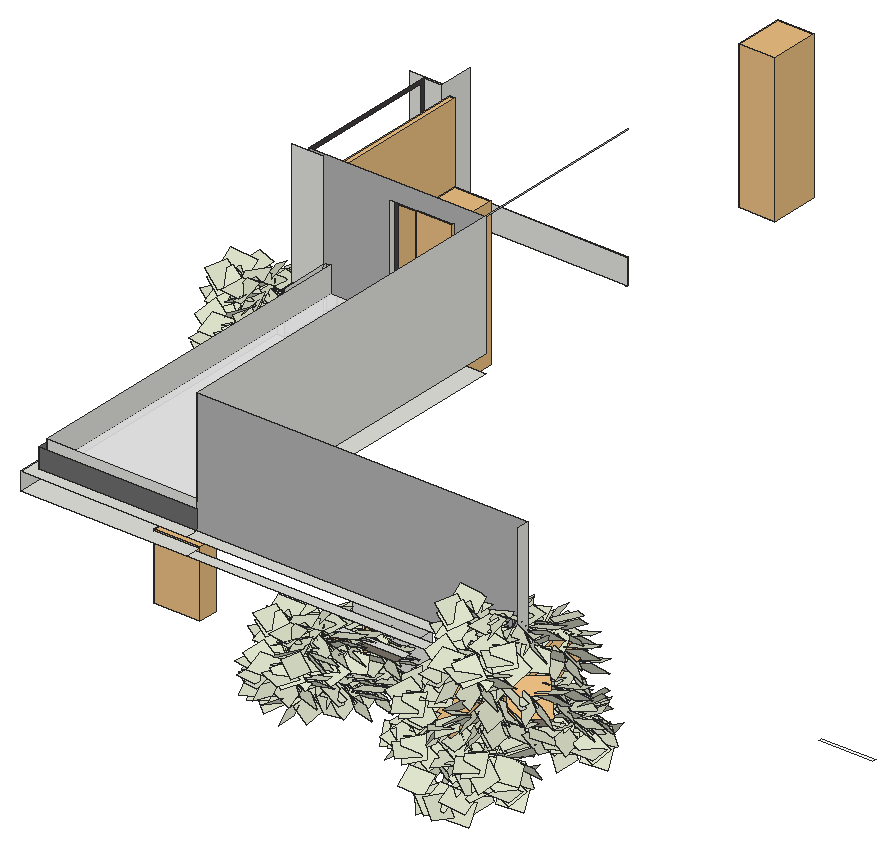
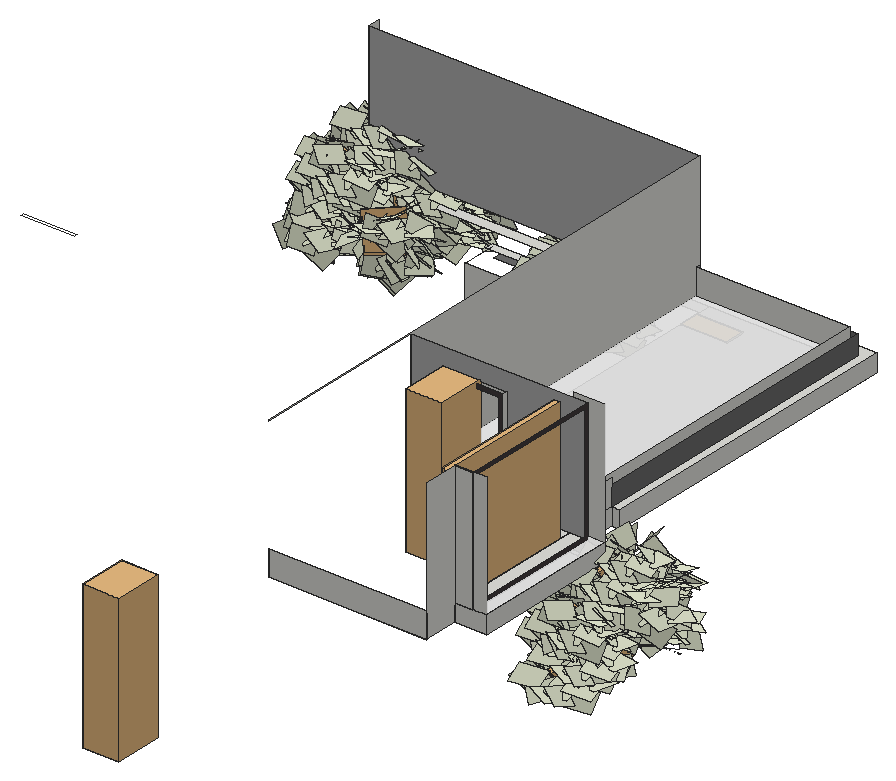
# SketchUp Ruby script. Lengths in inches.
U = 1.inch
M = Sketchup.active_model
def pt(a) = Geom::Point3d.new(a.map { |v| v * U })
def face(e, loops, mat)
  f = e.add_face(loops[0].map { |a| pt(a) })
  loops[1..].each { |l| e.add_face(l.map { |a| pt(a) }).erase! }
  f.material = f.back_material = mat if mat
  f
end
# faces: each face lists its corners as indices into pts; further lists are holes
def faces(e, pts, list, mat = nil) = list.each { |f| face(e, (f[0].is_a?(Array) ? f : [f]).map { |l| l.map { |i| pts[i] } }, mat) }
# xy, xz, yz: faces in a plane at the given z, y or x. An outline is a flat list of corners, or four numbers for a rectangle; further outlines are holes
def ring(l) = l.size == 4 ? [[l[0], l[1]], [l[2], l[1]], [l[2], l[3]], [l[0], l[3]]] : l.each_slice(2).to_a
def flat(e, list, mat, &to3) = list.each { |f| face(e, (f[0].is_a?(Array) ? f : [f]).map { |l| ring(l).map { |u, v| to3.(u, v) } }, mat) }
def xy(e, z, list, mat = nil) = flat(e, list, mat) { |x, y| [x, y, z] }
def xz(e, y, list, mat = nil) = flat(e, list, mat) { |x, z| [x, y, z] }
def yz(e, x, list, mat = nil) = flat(e, list, mat) { |y, z| [x, y, z] }
def lines(e, pts, list) = list.each { |a, b| e.add_line(pt(pts[a]), pt(pts[b])) }
# prism: a flat outline (further loops are holes) pulled along v
def prism(e, loops, v, mat = nil)
  f = face(e, loops, mat); d = Geom::Vector3d.new(v.map { |x| x * U })
  f.pushpull(f.normal.samedirection?(d) ? d.length : -d.length)
end
def box(e, o, s, mat = nil) = prism(e, [[o, [o[0] + s[0], o[1], o[2]], [o[0] + s[0], o[1] + s[1], o[2]], [o[0], o[1] + s[1], o[2]]]], [0, 0, s[2]], mat)
def at(x, y, z, deg = 0) = Geom::Transformation.translation(pt([x, y, z])) * Geom::Transformation.rotation(ORIGIN, Z_AXIS, deg.degrees)
def axes(o, x, y, z) = Geom::Transformation.new([*x, 0, *y, 0, *z, 0, *pt(o).to_a, 1])
def part(name) = M.definitions.add(name)
# library, detail: a bought-in or finely detailed component or shape, given as its bounding box
def library(name, o, s) = part(name).tap { |d| box(d.entities, o, s) }
def detail(e, o, s) = box(e.add_group.entities, o, s)
def put(e, d, t, mat = nil) = e.add_instance(d, t).tap { |i| i.material = mat if mat }
def group(e, t, mat = nil) = e.add_group.tap { |g| g.transformation = t; g.material = mat if mat }.entities
root = M.entities
M.materials.add("Celtis_australis_s cópia1").color = [224, 229, 205]
M.materials.add("Niraj_Hair_Dark").color = [109, 109, 109]
M.materials.add("Niraj_Hair_Gray").color = [178, 178, 178]
M.materials.add("Tendaggio").color = [239, 239, 239]
M.materials["Tendaggio"].alpha = 0.9
M.materials.add("[Asphalt New]").color = [67, 60, 62]
M.materials.add("[CoolGray4]").color = [225, 226, 230]
M.materials["[CoolGray4]"].alpha = 0.26
M.materials.add("bark_cherry").color = [99, 76, 62]
c1 = part("leaf1\#1")
p = [[1.6,6.78,0.04],[-9.34,-4.04,0.02],[2.67,-16.2,2.05],[13.62,-5.38,2.07]]
faces(c1.entities,p,[[0,1,2,3]],"Celtis_australis_s cópia1")
c2 = part("leaf_group1\#1")
put(c2.entities,c1,axes([-0.06,3.68,7.3125],[0.53029,-0.80282,-0.27253],[0.82812,0.42159,0.36943],[-0.18168,-0.42159,0.8884]))
put(c2.entities,c1,axes([6.4375,-3.58,5.23],[1,0,0],[0,0.98927,0.14608],[0,-0.14608,0.98927]))
put(c2.entities,c1,axes([-0.99,3.68,1.22],[0.57591,-0.80282,0.15431],[0.36532,0.42159,0.82994],[-0.73135,-0.42159,0.53609]))
put(c2.entities,c1,axes([18.71,8.59,4.39],[0.33053,0.77491,0.53877],[-0.79988,-0.073,0.5957],[0.50094,-0.62785,0.5957]))
put(c2.entities,c1,axes([13.16,0.76,0.89],[0.89618,0.3501,0.27256],[-0.44248,0.65988,0.60727],[0.03275,-0.66482,0.74628]))
put(c2.entities,c1,axes([4.53,7.98,7.3125],[-0.1927,0.94265,-0.27253],[0.88368,0.28746,0.36943],[-0.42658,0.16964,0.8884]))
put(c2.entities,c1,axes([12.46,21.28,7.16],[0.85019,0.38493,0.35918],[0.30538,-0.91629,0.25914],[-0.42887,0.11063,0.89657]))
put(c2.entities,c1,axes([6.53,15.18,2.59],[0.70711,0.70711,0],[0.5,-0.5,0.70711],[-0.5,0.5,0.70711]))
put(c2.entities,c1,axes([-3.17,8.15,3.46],[-0.03719,0.74973,0.66069],[0.94096,-0.19634,0.27576],[-0.33647,-0.63194,0.69817]))
put(c2.entities,c1,axes([23.03,17.79,4.39],[0.78166,-0.31422,0.53877],[-0.61722,-0.51398,0.5957],[-0.08973,0.79818,0.5957]))
put(c2.entities,c1,axes([14.78,21.52,3.21],[0.67246,-0.04394,0.73882],[-0.28657,-0.93583,0.20517],[-0.6824,0.3497,0.64191]))
put(c2.entities,c1,axes([10.37,-1.8125,9],[0.99279,-0.06448,-0.101],[0.11527,0.74421,0.65792],[0.03275,-0.66482,0.74628]))
put(c2.entities,c1,axes([1.45,16.1875,2.9375],[-0.2106,-0.86579,-0.45394],[0.96054,-0.26957,0.06852],[-0.18168,-0.42159,0.8884]))
c3 = library("branch1\#2",[0,0,0],[33.4,33.29,108.01])
c4 = part("branch2\#1")
p = [[13.74,0.36,0.5],[11.5,11.3125,10.98],[14.125,0.95,0],[14.97,0.95,0.19],[12.12,10.6875,11.67],[15.1,0.36,0.82],
  [11.05,10.4375,11.49],[14.34,0,1.01],[6.08,18.54,23.51],[6.83,18.32,23.89],[6.09,17.93,24.13],[3.27,29.37,34],
  [3.27,29.68,33.56],[3.73,29.59,33.82],[0,43.16,40.74],[0,43.16,40.75],[0.01,43.16,40.75],[5.59,23.2,32.77],
  [4.65,30.48,39.08],[1.92,39.79,43.02],[5.09,28.47,41.41]]
faces(c4.entities,p,[[0,1,2],[2,1,3],[3,4,5],[3,1,4],[6,0,7],[0,6,1],[5,6,7],[6,5,4],
  [6,8,1],[1,9,4],[9,1,8],[8,6,10],[4,10,6],[10,4,9],[10,11,8],[8,12,9],
  [12,8,11],[10,9,11],[13,11,9],[13,9,12],[14,12,11,15],[12,14,16,13],[13,16,15,11]],"bark_cherry")
lines(c4.entities,p,[[17,18],[11,19],[20,17],[17,10]])
c5 = part("branch3")
p = [[6.085,7.082,2.644],[4.083,0.001,0],[4.08,0.002,0.001],[5.841,7.141,2.739],[4.083,0,0.004],[6.032,7.035,2.901],
  [8.234,14.378,3.666],[10.055,21.673,1.937],[8.611,14.241,3.496],[10.247,21.661,2.456],[9.737,21.9,2.346],[9.715,21.803,2.365],
  [12.357,28.999,2.225],[12.894,28.763,2.608],[12.761,28.844,2.204],[10.064,22.087,2.083],[10.362,21.9,2.346],[5.434,16.028,3.111],
  [10.04,22.14,2.516],[12.239,29.014,2.642],[8.553,14.232,3.928],[5.628,15.927,3.273],[5.444,16.098,3.367],[12.571,28.869,2.879],
  [0.628,10.534,6.01],[0.625,10.536,6.008],[0.625,10.537,6.012],[6.135,9.846,4.735],[0.003,10.534,6.01],[0,10.537,6.012],
  [1.761,10.232,4.093],[4.16,5.476,4.049],[3.718,5.459,5.543],[3.205,0.783,1.919]]
faces(c5.entities,p,[[0,1,2,3],[3,2,4,5],[1,0,5,4],[6,7,8],[9,8,7],[7,6,10,11],[12,7,11],[13,7,14],
  [14,7,12],[13,9,7],[15,16,17],[15,17,18],[12,11,19],[20,10,6],[10,20,9,11],[21,17,16],
  [21,16,22],[18,22,16],[9,19,11],[8,9,20],[22,18,17],[9,13,23],[19,9,23],[0,8,5],
  [3,6,0],[8,0,6],[3,5,6],[20,5,8],[20,6,5],[21,24,25,17],[26,22,17,25],[22,26,24,21]],"bark_cherry")
lines(c5.entities,p,[[27,20],[28,29],[17,30],[27,31],[32,27],[5,33]])
c6 = part("branch1\#1")
p = [[23.875,19.65,51.47],[23.47,20.4,51.62],[21.1,21.64,19.5],[21.93,21.1875,19.92],[21.95,22.18,19.69],[26.48,9.62,42.86],
  [30.79,16.22,49.68],[31.01,4.77,55.38],[31.01,0,68.57],[9.91,24.21,59.69],[9.92,24.21,59.7],[24,20.54,51.64],
  [12.85,4.92,53.79],[26.1,8.92,42.74],[31.84,25.13,88.91],[31.84,25.13,106.45],[30.18,33.29,93.95],[30.18,25.42,69.53],
  [0,6.37,81.52],[11.1,10.75,77.87]]
lines(c6.entities,p,[[0,1],[2,3],[3,4],[5,6],[7,8],[9,10],[1,11],[11,0],[12,13],[4,2],[14,15],[16,17],
  [18,19]])
detail(c6.entities,[5.26,2.24,0],[28.14,24.14,108.01])
c7 = library("Plane01\#1",[-62.23,-4.43,-95.54],[61.02,8.86,95.65])
c8 = library("Tenda",[0,0,0],[9.09,66.93,111.26])
c9 = library("fronceur+aubin+blanc+(3)",[-47.99,-0.29,1.66],[95.37,4.84,114.09])
xy(root,173.7,[[944.67,187.625,980.63,190.375]],"[CoolGray4]")
xy(root,191.59,[[691.32,91.1875,742.03,96.6875]],"Niraj_Hair_Dark")
xy(root,195.13,[[541.86,336.16,580.61,341.53]])
xy(root,195.52,[[686.21,91.1875,747.21,96.6875]])
xy(root,207.01,[[494.79,89.375,494.79,301.21,500.29,301.21,500.29,333.01,479.54,333.01,479.54,430.89,485.73,430.89,485.73,336.16,605.23,336.16,605.23,89.375],[605.23,89.375,823.9,96.6875],[485.73,336.16,500.29,430.89],[500.29,454.11,605.23,454.18]])
xy(root,218.5625,[[494.79,89.375,605.23,89.375,605.23,97.6875,500.29,97.6875,500.29,301.21,494.79,301.21],[605.23,89.375,823.9,97.6875],[488.54,336.16,500.29,430.89]])
xy(root,218.5625,[[503.33,100.3125,605.23,100.3125,605.23,336.16,580.61,336.16,580.61,339.47,541.86,339.47,541.86,336.16,488.54,336.16,488.54,430.89,479.54,430.89,479.54,333.01,500.29,333.01,500.29,335.4,503.33,335.4]],"Tendaggio")
xz(root,97.6875,[[500.29,218.5625,605.23,231.41]],"Niraj_Hair_Dark")
xz(root,97.6875,[[605.23,218.5625,823.9,300.47]],"Niraj_Hair_Gray")
xz(root,100.3125,[[503.33,218.5625,605.23,235.75]])
xz(root,113.9375,[[[834.53,162.82,860.28,188.57],[835.87,164.16,858.9375,187.23]]],"[Asphalt New]")
xz(root,113.9375,[[835.87,164.16,858.9375,187.23]],"[CoolGray4]")
xz(root,119.5,[[690.76,157.6,743.01,197.92]])
xz(root,301.21,[[494.79,207.01,500.29,218.5625]])
xz(root,333.01,[[479.54,207.01,500.29,218.5625],[479.54,218.5625,500.29,300.47]])
xz(root,335.4,[[500.29,218.5625,503.33,235.75]])
xz(root,336.16,[[488.54,218.5625,541.86,218.5625,541.86,287.65,580.61,287.65,580.61,218.5625,605.23,218.5625,605.23,299.625,488.54,299.625]],"Niraj_Hair_Gray")
xz(root,339.47,[[[541.86,218.5625,580.61,287.65],[544.51,221.21,577.96,285]]],"[Asphalt New]")
xz(root,430.89,[[479.54,207.01,500.29,218.5625],[479.54,218.5625,488.54,218.5625,488.54,299.625,500.29,299.625,500.29,300.47,479.54,300.47],[488.54,218.5625,500.29,299.625]])
xz(root,454.11,[[500.29,207.01,605.23,224.0625]])
xz(root,454.18,[[500.29,207.01,605.23,224.0625]])
yz(root,479.54,[[333.01,207.01,430.89,218.5625]])
yz(root,488.54,[[[336.16,218.5625,430.89,299.625],[338.54,220.95,428.5,297.24]]],"[Asphalt New]")
yz(root,494.79,[[89.375,207.01,301.21,218.5625]])
yz(root,500.29,[[301.21,207.01,333.01,218.5625],[336.16,207.01,430.89,218.5625],[430.89,207.01,454.11,299.625],[454.11,207.01,454.18,224.0625],[301.21,218.5625,333.01,235.75],
  [333.01,218.5625,335.4,235.75]])
yz(root,500.29,[[97.6875,218.5625,301.21,231.41]],"Niraj_Hair_Dark")
yz(root,503.33,[[100.3125,218.5625,335.4,235.75]])
yz(root,541.86,[[336.16,218.5625,339.47,287.65]])
yz(root,580.61,[[336.16,218.5625,339.47,287.65]],"[Asphalt New]")
yz(root,605.23,[[454.11,207.01,454.18,224.0625],[100.3125,218.5625,100.3125,235.75,97.6875,235.75,97.6875,300.47,454.11,300.47,454.11,299.625,336.16,299.625,336.16,218.5625]])
yz(root,823.9,[[89.375,218.5625,97.6875,300.47]])
p = [[743.01,96.6875,197.92],[743.01,119.5,197.92],[743.01,96.6875,157.6],[743.01,119.5,157.6],[690.76,96.6875,197.92],[690.76,119.5,197.92],
  [690.76,96.6875,157.6],[690.76,119.5,157.6],[472.19,322.9,213.64],[472.19,326.9,204.86],[471.05,313.38,210.83],[471.05,314.6,212.2],
  [471.73,322.89,207.53],[471.73,318.5,207.53],[471.73,316.66,204.86],[471.05,317.1,212.2],[705.56,71.08,201.25],[705.56,75.09,194.44],
  [704.41,61.57,199.07],[704.41,62.79,200.13],[705.09,71.08,196.51],[705.09,66.68,196.51],[705.09,64.85,194.44],[704.41,65.29,200.13],
  [465.37,367.86,175.4],[465.37,372.36,168.78],[464.08,357.16,173.28],[464.08,358.54,174.3125],[464.85,367.85,170.79],[464.85,362.91,170.79],
  [464.85,360.85,168.78],[464.08,361.35,174.3125]]
lines(root,p,[[0,1],[2,3],[4,5],[6,7],[8,9],[10,11],[12,13],[14,13],[15,11],[16,17],[18,19],[20,21],
  [22,21],[23,19],[24,25],[26,27],[28,29],[30,29],[31,27]])
put(root,c2,axes([472.09,349.22,169.9375],[0.53001,-0.70334,-0.12848],[0.71079,0.53562,0],[0.07732,-0.10261,0.88068]))
put(root,c3,axes([460.68,352.72,152.52],[0.43496,-0.31874,0.04505],[-0.24964,-0.28618,0.38548],[0.15157,0.24659,0.28123]))
put(root,c2,axes([440.37,314.79,170.27],[0.8327,-0.28672,-0.12848],[0.28976,0.84151,0],[0.12148,-0.04183,0.88068]))
put(root,c2,axes([447.5,394.25,165.95],[0.59551,-0.79027,-0.09672],[0.79864,0.60182,0],[0.08688,-0.11529,0.66298]))
put(root,c2,axes([660.23,88.625,166.46],[0.53023,-0.70334,-0.09885],[0.71078,0.53562,0.00096],[0.07578,-0.10261,0.68258]))
put(root,c2,axes([837.78,23.22,169.88],[-0.41131,0.78137,0.11126],[-0.78924,-0.4063,-0.06424],[-0.0056,-0.12835,0.88068]))
put(root,c4,axes([460.44,348.03,165.87],[0.26446,-0.63222,0],[-0.57063,-0.2387,-0.29503],[-0.19324,-0.08084,0.43916]))
put(root,c2,axes([792.98,114.66,173.33],[-0.04359,-0.87249,0.17019],[0.84765,0.01053,0.27108],[-0.26776,0.17537,0.83045]))
put(root,c4,axes([453.41,377.49,157],[0.39588,0.27856,-0.02127],[0.15584,-0.23409,-0.07417],[0.10636,-0.10805,0.25341]))
put(root,c5,axes([479.125,378.34,159.23],[-0.16853,0.67581,-0.04682],[-0.62427,-0.18244,-0.17343],[-0.26812,0,0.43323]))
put(root,c2,axes([705.45,97.41,167.38],[0.53001,-0.70334,-0.09956],[0.71079,0.53562,0],[0.07732,-0.10261,0.68247]))
put(root,c2,axes([456.68,362.41,171.38],[0.53001,-0.70334,-0.12848],[0.71079,0.53562,0],[0.07732,-0.10261,0.88068]))
put(root,c2,axes([458.03,374.4,165.26],[-0.28104,-0.95381,0.0711],[0.95882,-0.27434,0.04925],[-0.041,0.12241,0.66439]))
put(root,c3,axes([694.04,100.91,153.88],[0.43496,-0.31874,0.03491],[-0.24964,-0.28618,0.29872],[0.15157,0.24659,0.21794]))
put(root,c2,axes([673.73,62.98,167.64],[0.8327,-0.28672,-0.09956],[0.28976,0.84151,0],[0.12148,-0.04183,0.68247]))
put(root,c2,axes([842.14,38.76,171.66],[0.53183,0.70196,-0.12848],[-0.70939,0.53746,0],[0.07759,0.10241,0.88068]))
put(root,c4,axes([693.8,96.22,164.23],[0.26446,-0.63222,0],[-0.57063,-0.2387,-0.22863],[-0.19324,-0.08084,0.34033]))
put(root,c2,axes([690.04,110.6,168.5],[0.53001,-0.70334,-0.09956],[0.71079,0.53562,0],[0.07732,-0.10261,0.68247]))
put(root,c2,axes([797.49,100.59,173.27],[0.03764,0.88184,0.1142],[-0.86164,0.00793,0.22275],[0.21969,-0.11998,0.85407]))
put(root,c2,axes([820.06,40.99,178.51],[0.74921,0.45418,0.15655],[-0.41604,0.75843,-0.20928],[-0.24021,0.10299,0.85076]))
put(root,c2,axes([460.58,340.32,174.44],[0.53001,-0.70334,-0.12848],[0.71079,0.53562,0],[0.07732,-0.10261,0.88068]))
put(root,c2,axes([472.09,331.59,174.44],[0.53001,-0.70334,-0.12848],[0.71079,0.53562,0],[0.07732,-0.10261,0.88068]))
put(root,c2,axes([475.63,326.85,174.44],[0.53001,-0.70334,-0.12848],[-0.71079,-0.53562,0],[0.07732,-0.10261,0.88068]))
put(root,c3,axes([821.64,105.65,157],[-0.52875,-0.46238,0.03129],[0.31975,-0.32962,0.53241],[-0.2583,0.31925,0.35278]))
put(root,c2,axes([693.94,88.51,170.875],[0.53001,-0.70334,-0.09956],[0.71079,0.53562,0],[0.07732,-0.10261,0.68247]))
put(root,c2,axes([705.45,79.78,170.875],[0.53001,-0.70334,-0.09956],[0.71079,0.53562,0],[0.07732,-0.10261,0.68247]))
put(root,c2,axes([708.99,75.04,170.875],[0.53001,-0.70334,-0.09956],[-0.71079,-0.53562,0],[0.07732,-0.10261,0.68247]))
put(root,c2,axes([466.69,369.97,174.94],[0.53001,-0.70334,-0.12848],[0.71079,0.53562,0],[0.07732,-0.10261,0.88068]))
put(root,c2,axes([700.05,118.16,171.26],[0.53001,-0.70334,-0.09956],[0.71079,0.53562,0],[0.07732,-0.10261,0.68247]))
put(root,c2,axes([447.5,378.125,170.89],[0.59551,-0.79027,-0.09672],[0.79864,0.60182,0],[0.08688,-0.11529,0.66298]))
put(root,c6,axes([467.83,381.64,157.91],[-0.19674,0.14054,0.02551],[-0.11292,-0.18767,0.07321],[0.06856,0.05241,0.10778]))
put(root,c2,axes([668.56,88.625,195.48],[0.33028,-0.70334,-0.3363],[0.5516,0.53562,-0.34739],[0.61543,-0.10261,0.49184]))
put(root,c5,axes([448.66,350.93,159.7],[1,0,0],[0,1,0],[0,0,0.67]))
put(root,c2,axes([435.2,340.4375,206.2],[0.33028,-0.70334,-0.43397],[0.5516,0.53562,-0.44828],[0.61543,-0.10261,0.63468]))
put(root,c2,axes([786.82,126,206.9375],[0.33028,-0.70334,-0.43397],[0.5516,0.53562,-0.44828],[0.61543,-0.10261,0.63468]))
put(root,c2,axes([855.9375,91.05,178.45],[0.53183,0.70196,-0.12848],[-0.70939,0.53746,0],[0.07759,0.10241,0.88068]))
put(root,c5,axes([463.13,381.42,177.56],[-0.72608,-0.15932,-0.15831],[0.2243,0.07943,-0.49769],[0.17579,-0.75941,-0.01884]))
put(root,c4,axes([687.79,84.875,172.03],[0.66608,0.16114,0],[0.14545,-0.6012,-0.22863],[0.06937,-0.28676,0.47933]))
put(root,c2,axes([783.08,125.4,182.35],[-0.04359,-0.87249,0.17019],[0.84765,0.01053,0.27108],[-0.26776,0.17537,0.83045]))
put(root,c2,axes([773.25,67.875,180.65],[0.88068,0,-0.12848],[0,0.89,0],[0.12848,0,0.88068]))
put(root,c2,axes([801.57,65.55,180.65],[-0.88068,0,-0.12848],[0,-0.89,0],[-0.12848,0,0.88068]))
put(root,c2,axes([828.75,128.95,180.84],[-0.03841,-0.87984,-0.12848],[0.88915,-0.03882,0],[-0.0056,-0.12835,0.88068]))
put(root,c4,axes([454.43,336.6875,175.9375],[0.66608,0.16114,0],[0.14545,-0.6012,-0.29503],[0.06937,-0.28676,0.61854]))
put(root,c2,axes([821.15,100.65,180.12],[-0.41131,0.78137,0.11126],[-0.78924,-0.4063,-0.06424],[-0.0056,-0.12835,0.88068]))
put(root,c7,axes([605.84,106.43,207.57],[0.5,0,0],[0,-1.43153,0],[0,0,0.45937]))
put(root,c2,axes([789.17,37.93,181.91],[0.88059,0.0123,-0.12848],[-0.01243,0.88991,0],[0.12846,0.00179,0.88068]))
put(root,c3,axes([826.42,71.82,164.43],[-0.66136,0.25698,0.05927],[0.21982,0.44874,0.50721],[-0.0849,-0.28517,0.28909]))
put(root,c2,axes([690.04,122.94,179.11],[0.53001,-0.70334,-0.09956],[0.71079,0.53562,0],[0.07732,-0.10261,0.68247]))
put(root,c2,axes([700.39,110.6,180.14],[0.53001,-0.70334,-0.09956],[0.71079,0.53562,0],[0.07732,-0.10261,0.68247]))
put(root,c2,axes([685.6,59.14,180.34],[0.53023,-0.70334,-0.09885],[0.71078,0.53562,0.00096],[0.07578,-0.10261,0.68258]))
put(root,c2,axes([456.68,374.76,185.07],[0.53001,-0.70334,-0.12848],[0.71079,0.53562,0],[0.07732,-0.10261,0.88068]))
put(root,c2,axes([829.42,102.09,185.27],[0.86375,-0.17184,-0.12848],[0.17366,0.87289,0],[0.12601,-0.02507,0.88068]))
put(root,c2,axes([829.42,41.85,185.27],[0.86375,-0.17184,-0.12848],[0.17366,0.87289,0],[0.12601,-0.02507,0.88068]))
put(root,c2,axes([467.03,362.41,186.4],[0.53001,-0.70334,-0.12848],[0.71079,0.53562,0],[0.07732,-0.10261,0.88068]))
put(root,c2,axes([452.24,310.95,186.66],[0.53023,-0.70334,-0.12755],[0.71078,0.53562,0.00124],[0.07578,-0.10261,0.88081]))
put(root,c2,axes([667.26,93.79,182.93],[0.16522,-0.86518,-0.09885],[0.87423,0.16677,0.00096],[0.02269,-0.12552,0.68258]))
put(root,c2,axes([807.76,45.49,193.3],[0.87255,-0.07903,0.15655],[0.1152,0.85734,-0.20928],[-0.13223,0.22544,0.85076]))
put(root,c2,axes([840.35,111.99,188.89],[-0.03841,-0.87984,-0.12848],[0.88915,-0.03882,0],[-0.0056,-0.12835,0.88068]))
put(root,c2,axes([690.45,50.61,184.95],[0.80207,0.36403,-0.09885],[-0.36766,0.81051,0.00096],[0.11667,0.05157,0.68258]))
put(root,c2,axes([690.31,104.82,185.66],[0.84485,-0.24865,-0.09956],[0.25128,0.85379,0],[0.12325,-0.03627,0.68247]))
put(root,c2,axes([433.9,345.6,189.99],[0.16522,-0.86518,-0.12755],[0.87423,0.16677,0.00124],[0.02269,-0.12552,0.88081]))
put(root,c4,axes([694.78,95.28,174.43],[0.19838,-0.63222,-0.13553],[-0.62314,-0.2387,0.12094],[0.14547,-0.08084,0.35432]))
put(root,c2,axes([773.25,75.16,190.22],[0.88068,0,-0.12848],[0,0.89,0],[0.12848,0,0.88068]))
put(root,c2,axes([837.91,80.65,190.29],[0.53183,0.70196,-0.12848],[-0.70939,0.53746,0],[0.07759,0.10241,0.88068]))
put(root,c3,axes([818.95,108.73,189.57],[-0.4587,-0.54131,0.05927],[0.35246,-0.35421,-0.50721],[0.24186,-0.1733,0.28909]))
put(root,c2,axes([839.31,93.1,190.39],[-0.4192,-0.77451,-0.12848],[0.78271,-0.42363,0],[-0.06115,-0.11299,0.88068]))
put(root,c2,axes([801.18,112.67,190.92],[-0.41131,0.78137,0.11126],[-0.78924,-0.4063,-0.06424],[-0.0056,-0.12835,0.88068]))
put(root,c2,axes([801.18,100.65,190.92],[-0.41131,0.78137,0.11126],[-0.78924,-0.4063,-0.06424],[-0.0056,-0.12835,0.88068]))
put(root,c2,axes([700.67,71.65,187.97],[0.87731,0.07848,-0.09885],[-0.07912,0.88648,0.00096],[0.12716,0.01012,0.68258]))
put(root,c2,axes([796.51,56.53,192.45],[0.53001,-0.70334,-0.12848],[0.71079,0.53562,0],[0.07732,-0.10261,0.88068]))
put(root,c2,axes([457.09,302.42,192.61],[0.80207,0.36403,-0.12755],[-0.36766,0.81051,0.00124],[0.11667,0.05157,0.88081]))
put(root,c2,axes([456.95,356.63,193.52],[0.84485,-0.24865,-0.12848],[0.25128,0.85379,0],[0.12325,-0.03627,0.88068]))
put(root,c4,axes([461.42,347.09,179.04],[0.19838,-0.63222,-0.17489],[-0.62314,-0.2387,0.15606],[0.14547,-0.08084,0.45722]))
put(root,c4,axes([706.14,84.25,179.4375],[-0.53333,-0.02085,-0.1671],[-0.03241,0.3542,0.03557],[-0.17665,-0.07371,0.34411]))
put(root,c2,axes([689.65,94.58,191.52],[0.53001,-0.70334,-0.09956],[0.71079,0.53562,0],[0.07732,-0.10261,0.68247]))
put(root,c4,axes([694.91,79.66,182.32],[0.35233,0.24792,-0.02189],[0.1387,-0.20834,-0.07635],[0.09466,-0.09617,0.26086]))
put(root,c5,axes([717.8,80.41,184.61],[-0.14999,0.60147,-0.0482],[-0.5556,-0.16237,-0.17853],[-0.23862,0,0.44597]))
put(root,c2,axes([467.31,323.46,196.5],[0.87731,0.07848,-0.12755],[-0.07912,0.88648,0.00124],[0.12716,0.01012,0.88081]))
put(root,c2,axes([699.02,76.91,190.82],[-0.25013,-0.84889,0.07319],[0.85335,-0.24416,0.0507],[-0.03649,0.10895,0.68393]))
put(root,c4,axes([472.78,336.06,185.49],[-0.53333,-0.02085,-0.21563],[-0.03241,0.3542,0.0459],[-0.17665,-0.07371,0.44405]))
put(root,c8,axes([571.04,588.5,182.78],[0,3.55421,0],[0.35907,0,0],[0,0,0.87048]))
put(root,c2,axes([689.65,80.22,196.61],[0.53001,-0.70334,-0.09956],[0.71079,0.53562,0],[0.07732,-0.10261,0.68247]))
put(root,c6,axes([707.74,83.35,183.25],[-0.1751,0.12508,0.02626],[-0.1005,-0.16702,0.07536],[0.06102,0.04664,0.11094]))
put(root,c2,axes([829.14,75.04,200.96],[0.53001,-0.70334,-0.12848],[-0.71079,-0.53562,0],[0.07732,-0.10261,0.88068]))
put(root,c2,axes([832.26,75.04,200.96],[0.53001,-0.70334,-0.12848],[-0.71079,-0.53562,0],[0.07732,-0.10261,0.88068]))
put(root,c2,axes([456.29,346.39,201.09],[0.53001,-0.70334,-0.12848],[0.71079,0.53562,0],[0.07732,-0.10261,0.88068]))
put(root,c2,axes([782.86,48.86,201.46],[0.86375,-0.17184,-0.12848],[0.17366,0.87289,0],[0.12601,-0.02507,0.88068]))
put(root,c4,axes([461.55,331.47,189.21],[0.35233,0.24792,-0.02825],[0.1387,-0.20834,-0.09852],[0.09466,-0.09617,0.33662]))
put(root,c5,axes([484.4375,332.22,192.17],[-0.14999,0.60147,-0.06219],[-0.5556,-0.16237,-0.23038],[-0.23862,0,0.57549]))
put(root,c2,axes([465.66,328.72,200.18],[-0.25013,-0.84889,0.09445],[0.85335,-0.24416,0.06542],[-0.03649,0.10895,0.88255]))
put(root,c2,axes([781,127.84,202.625],[-0.03841,-0.87984,-0.12848],[0.88915,-0.03882,0],[-0.0056,-0.12835,0.88068]))
put(root,c5,axes([690.68,56.02,185.1],[0.89,0,0],[0,0.89,0],[0,0,0.6897]))
put(root,c5,axes([703.56,83.16,203.48],[-0.64621,-0.1418,-0.16297],[0.19963,0.07069,-0.51232],[0.15645,-0.67588,-0.0194]))
put(root,c2,axes([780.38,88.625,204.4375],[0.53023,-0.70334,-0.12755],[0.71078,0.53562,0.00124],[0.07578,-0.10261,0.88081]))
put(root,c2,axes([825.6,97.41,205.63],[0.53001,-0.70334,-0.12848],[0.71079,0.53562,0],[0.07732,-0.10261,0.88068]))
put(root,c3,axes([814.19,100.91,188.21],[0.43496,-0.31874,0.04505],[-0.24964,-0.28618,0.38548],[0.15157,0.24659,0.28123]))
put(root,c2,axes([793.875,62.98,205.96],[0.8327,-0.28672,-0.12848],[0.28976,0.84151,0],[0.12148,-0.04183,0.88068]))
put(root,c4,axes([813.95,96.22,201.5625],[0.26446,-0.63222,0],[-0.57063,-0.2387,-0.29503],[-0.19324,-0.08084,0.43916]))
put(root,c2,axes([810.19,110.6,207.08],[0.53001,-0.70334,-0.12848],[0.71079,0.53562,0],[0.07732,-0.10261,0.88068]))
put(root,c2,axes([456.29,332.04,207.65],[0.53001,-0.70334,-0.12848],[0.71079,0.53562,0],[0.07732,-0.10261,0.88068]))
put(root,c6,axes([474.38,335.16,190.41],[-0.1751,0.12508,0.03388],[-0.1005,-0.16702,0.09725],[0.06102,0.04664,0.14316]))
put(root,c8,axes([560.13,334.76,191.27],[0,3.55421,0],[0.35907,0,0],[0,0,0.87048]))
put(root,c2,axes([814.09,88.51,210.14],[0.53001,-0.70334,-0.12848],[0.71079,0.53562,0],[0.07732,-0.10261,0.88068]))
put(root,c2,axes([825.6,79.78,210.14],[0.53001,-0.70334,-0.12848],[0.71079,0.53562,0],[0.07732,-0.10261,0.88068]))
put(root,c2,axes([829.14,75.04,210.14],[0.53001,-0.70334,-0.12848],[-0.71079,-0.53562,0],[0.07732,-0.10261,0.88068]))
put(root,c5,axes([457.32,307.83,192.79],[0.89,0,0],[0,0.89,0],[0,0,0.89]))
put(root,c2,axes([820.2,118.16,210.64],[0.53001,-0.70334,-0.12848],[0.71079,0.53562,0],[0.07732,-0.10261,0.88068]))
put(root,c5,axes([470.2,334.97,216.51],[-0.64621,-0.1418,-0.21029],[0.19963,0.07069,-0.66111],[0.15645,-0.67588,-0.02503]))
put(root,c2,axes([788.71,88.625,241.89],[0.33028,-0.70334,-0.43397],[0.5516,0.53562,-0.44828],[0.61543,-0.10261,0.63468]))
put(root,c4,axes([807.94,84.875,211.63],[0.66608,0.16114,0],[0.14545,-0.6012,-0.29503],[0.06937,-0.28676,0.61854]))
put(root,c2,axes([810.19,122.94,220.76],[0.53001,-0.70334,-0.12848],[0.71079,0.53562,0],[0.07732,-0.10261,0.88068]))
put(root,c2,axes([820.54,110.6,222.09],[0.53001,-0.70334,-0.12848],[0.71079,0.53562,0],[0.07732,-0.10261,0.88068]))
put(root,c2,axes([805.75,59.14,222.35],[0.53023,-0.70334,-0.12755],[0.71078,0.53562,0.00124],[0.07578,-0.10261,0.88081]))
put(root,c2,axes([787.41,93.79,225.6875],[0.16522,-0.86518,-0.12755],[0.87423,0.16677,0.00124],[0.02269,-0.12552,0.88081]))
put(root,c2,axes([810.6,50.61,228.3],[0.80207,0.36403,-0.12755],[-0.36766,0.81051,0.00124],[0.11667,0.05157,0.88081]))
put(root,c2,axes([810.46,104.82,229.21],[0.84485,-0.24865,-0.12848],[0.25128,0.85379,0],[0.12325,-0.03627,0.88068]))
put(root,c9,axes([505.98,383.9,210.48],[0,-0.97493,0],[0.73,0,0],[0,0,0.73]))
put(root,c4,axes([814.93,95.28,214.73],[0.19838,-0.63222,-0.17489],[-0.62314,-0.2387,0.15606],[0.14547,-0.08084,0.45722]))
put(root,c2,axes([820.82,71.65,232.2],[0.87731,0.07848,-0.12755],[-0.07912,0.88648,0.00124],[0.12716,0.01012,0.88081]))
put(root,c4,axes([826.29,84.25,221.18],[-0.53333,-0.02085,-0.21563],[-0.03241,0.3542,0.0459],[-0.17665,-0.07371,0.44405]))
put(root,c2,axes([809.8,94.58,236.78],[0.53001,-0.70334,-0.12848],[0.71079,0.53562,0],[0.07732,-0.10261,0.88068]))
